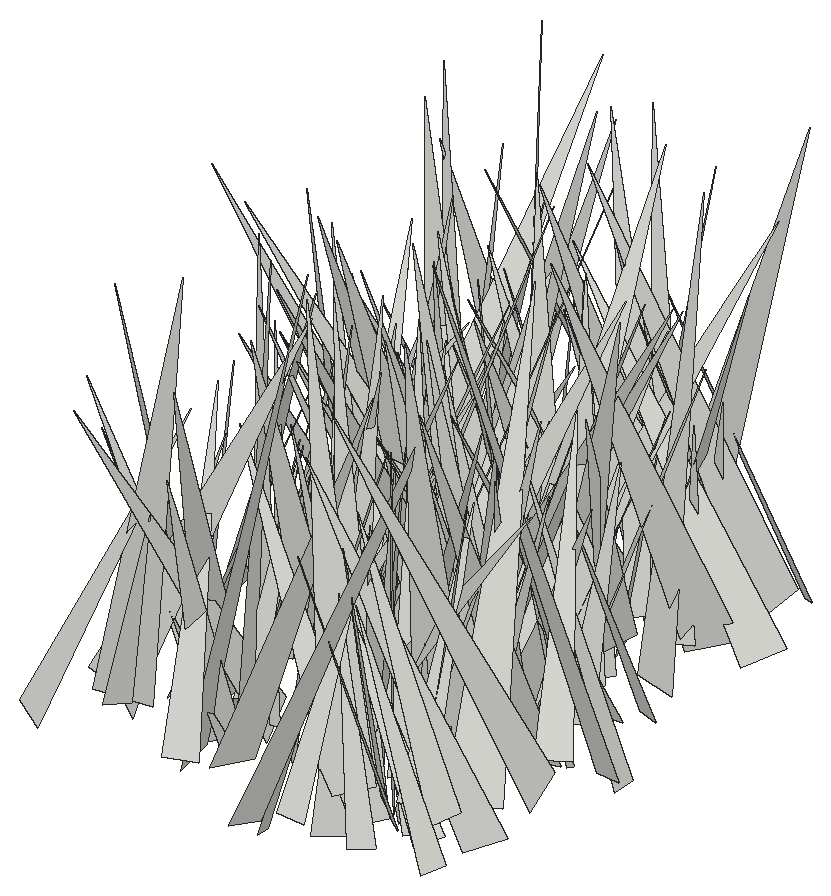
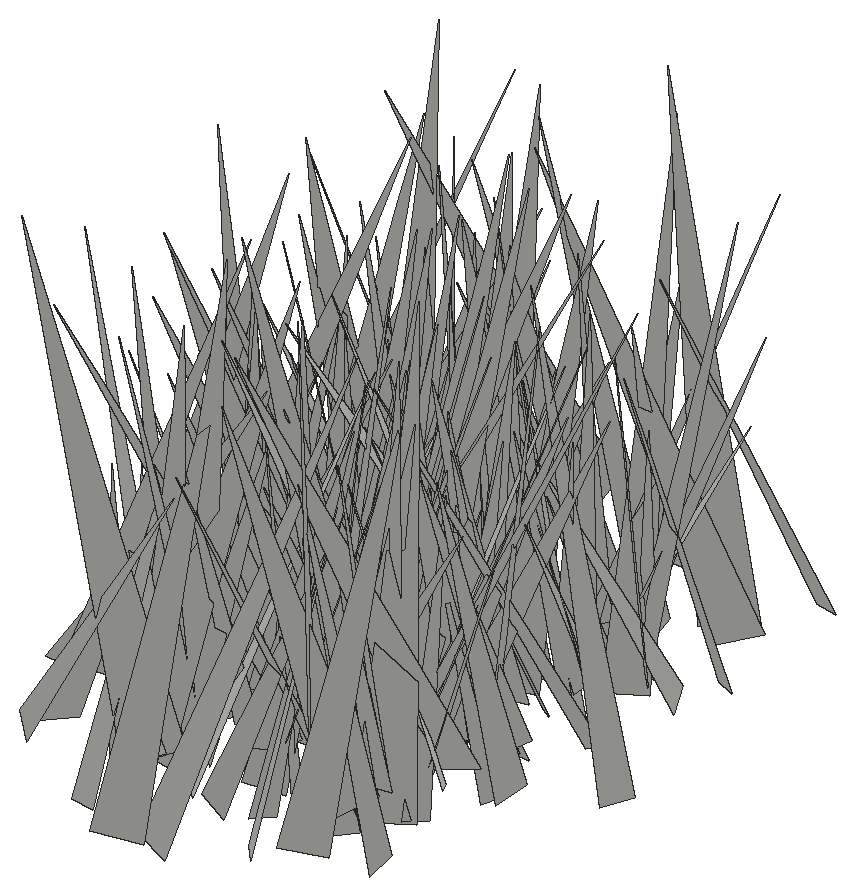
# SketchUp Ruby script. Lengths in inches.
U = 1.inch
M = Sketchup.active_model
def pt(a) = Geom::Point3d.new(a.map { |v| v * U })
def face(e, loops, mat)
  f = e.add_face(loops[0].map { |a| pt(a) })
  loops[1..].each { |l| e.add_face(l.map { |a| pt(a) }).erase! }
  f.material = f.back_material = mat if mat
  f
end
# faces: each face lists its corners as indices into pts; further lists are holes
def faces(e, pts, list, mat = nil) = list.each { |f| face(e, (f[0].is_a?(Array) ? f : [f]).map { |l| l.map { |i| pts[i] } }, mat) }
# xy, xz, yz: faces in a plane at the given z, y or x. An outline is a flat list of corners, or four numbers for a rectangle; further outlines are holes
def ring(l) = l.size == 4 ? [[l[0], l[1]], [l[2], l[1]], [l[2], l[3]], [l[0], l[3]]] : l.each_slice(2).to_a
def flat(e, list, mat, &to3) = list.each { |f| face(e, (f[0].is_a?(Array) ? f : [f]).map { |l| ring(l).map { |u, v| to3.(u, v) } }, mat) }
def xy(e, z, list, mat = nil) = flat(e, list, mat) { |x, y| [x, y, z] }
def xz(e, y, list, mat = nil) = flat(e, list, mat) { |x, z| [x, y, z] }
def yz(e, x, list, mat = nil) = flat(e, list, mat) { |y, z| [x, y, z] }
def lines(e, pts, list) = list.each { |a, b| e.add_line(pt(pts[a]), pt(pts[b])) }
# prism: a flat outline (further loops are holes) pulled along v
def prism(e, loops, v, mat = nil)
  f = face(e, loops, mat); d = Geom::Vector3d.new(v.map { |x| x * U })
  f.pushpull(f.normal.samedirection?(d) ? d.length : -d.length)
end
def box(e, o, s, mat = nil) = prism(e, [[o, [o[0] + s[0], o[1], o[2]], [o[0] + s[0], o[1] + s[1], o[2]], [o[0], o[1] + s[1], o[2]]]], [0, 0, s[2]], mat)
def at(x, y, z, deg = 0) = Geom::Transformation.translation(pt([x, y, z])) * Geom::Transformation.rotation(ORIGIN, Z_AXIS, deg.degrees)
def axes(o, x, y, z) = Geom::Transformation.new([*x, 0, *y, 0, *z, 0, *pt(o).to_a, 1])
def part(name) = M.definitions.add(name)
# library, detail: a bought-in or finely detailed component or shape, given as its bounding box
def library(name, o, s) = part(name).tap { |d| box(d.entities, o, s) }
def detail(e, o, s) = box(e.add_group.entities, o, s)
def put(e, d, t, mat = nil) = e.add_instance(d, t).tap { |i| i.material = mat if mat }
def group(e, t, mat = nil) = e.add_group.tap { |g| g.transformation = t; g.material = mat if mat }.entities
root = M.entities
c1 = part("fur_instance\#9")
p = [[0.8125,0,1.79],[0.67,-0.02,1.48],[0,-0.11,0],[0,0.11,0]]
faces(c1.entities,p,[[0,1,2,3]])
put(root,c1,axes([126.4,82.98,-27.1],[-4.21104,-1.2398,0.43934],[-1.31531,3.95873,-1.43574],[-0.00925,1.50143,4.14832]))
put(root,c1,axes([122.02,80.37,-28.22],[7.393,0.04175,0.28729],[0.1077,-7.1937,-1.72622],[-0.26959,-1.72907,7.18877]))
put(root,c1,axes([126.64,73.74,-27.1],[-5.33847,-0.05884,0.40473],[-0.0096,5.31499,0.64603],[0.40887,-0.64342,5.29956]))
put(root,c1,axes([125.85,74.4,-27.1],[-3.47477,-5.64058,1.59223],[-5.83486,3.50381,-0.32112],[0.55295,1.52727,6.61718]))
put(root,c1,axes([123.08,69.83,-27.1],[2.64419,5.03318,0.33977],[4.95036,-2.51506,-1.26831],[0.97076,-0.88412,5.54221]))
put(root,c1,axes([124.5,76.02,-27.1],[3.53151,3.08583,1.68165],[3.37882,-3.63698,-0.42174],[-0.96639,-1.43941,4.67077]))
put(root,c1,axes([123.76,73.4375,-28.22],[2.7927,4.03544,0.85961],[4.11922,-2.66751,-0.85986],[0.23622,-1.19268,4.83163]))
put(root,c1,axes([124.58,81.87,-28.22],[5.08359,-0.28901,1.82683],[-0.68576,-5.25683,1.07667],[-1.71772,1.24337,4.97667]))
put(root,c1,axes([127.85,83.42,-28.22],[-8.04638,-2.10125,0.20494],[-2.02323,7.90531,1.61682],[0.60315,-1.51404,8.15753]))
put(root,c1,axes([124.33,74.79,-28.22],[4.4552,2.25801,0.37031],[2.04407,-4.29173,1.57715],[-1.02836,1.2518,4.7392]))
put(root,c1,axes([127.79,73.02,-28.22],[-4.47703,-2.46915,0.00102],[-2.34184,4.24552,-1.62229],[-0.78262,1.42103,4.84857]))
put(root,c1,axes([125.86,81.34,-28.22],[-6.04607,-3.24149,2.31572],[-3.3744,6.40425,0.15438],[2.11738,0.95032,6.85845]))
put(root,c1,axes([125.81,76.18,-28.22],[3.59429,3.23742,0.8797],[2.57384,-3.488,2.32011],[-2.15177,1.23558,4.24464]))
put(root,c1,axes([126.67,76.94,-27.1],[1.26657,4.59176,1.22685],[4.36989,-1.62436,1.56816],[-1.86909,-0.68616,4.4977]))
put(root,c1,axes([126.86,81.64,-27.1],[0.11807,-5.18176,0.38422],[-4.95689,-0.22756,-1.54584],[-1.55804,0.33133,4.94722]))
put(root,c1,axes([125.82,89.55,-27.1],[3.87648,-5.20572,1.47803],[-5.00062,-4.14086,-1.46909],[-2.0683,0.2548,6.32205]))
put(root,c1,axes([124.22,78.45,-27.1],[2.61371,2.45973,0.53308],[2.49517,-2.43181,-1.01309],[0.32949,-1.09634,3.44317]))
put(root,c1,axes([124.6875,71.85,-27.1],[2.97768,-2.23657,0.59018],[-2.29034,-2.98547,0.24174],[-0.32391,0.5494,3.71623]))
put(root,c1,axes([124.91,81.26,-27.1],[3.82826,-1.89723,1.31218],[-2.241,-3.66166,1.2438],[-0.54703,1.72325,4.08754]))
put(root,c1,axes([127.42,75.15,-28.22],[1.80048,6.74236,1.9451],[6.61582,-2.30046,1.85022],[-2.33959,-1.31645,6.72888]))
put(root,c1,axes([125.53,77.95,-27.1],[4.20313,-0.16718,1.34956],[-0.39887,-4.34286,0.70427],[-1.30006,0.79192,4.14708]))
put(root,c1,axes([127.31,83.125,-28.22],[1.43774,-5.64122,0.58152],[-5.34924,-1.54822,-1.79367],[-1.88339,0.09091,5.53834]))
put(root,c1,axes([125.81,74.35,-28.22],[0.22689,-3.51122,0.97081],[-3.62685,-0.12635,0.39066],[0.3422,0.98893,3.49679]))
put(root,c1,axes([124.82,82.47,-28.22],[3.6641,-0.22277,0.06955],[-0.2117,-3.63329,-0.48425],[-0.09821,-0.47926,3.63879]))
put(root,c1,axes([126.34,85.27,-28.22],[-4.81324,5.46383,3.73935],[6.29264,5.21276,0.48307],[2.05886,-3.15867,7.26549]))
put(root,c1,axes([126.35,75.01,-28.22],[3.32895,2.2471,0.95718],[1.81279,-3.35751,1.57751],[-1.63691,0.85163,3.69362]))
put(root,c1,axes([126.71,84.79,-27.1],[3.29752,4.92899,1.52703],[4.76096,-3.60504,1.35547],[-1.98997,-0.45731,5.77332]))
put(root,c1,axes([124.9,87.24,-28.22],[5.83146,1.27805,1.15338],[1.33487,-5.92923,-0.17895],[-1.08712,-0.42484,5.96719]))
put(root,c1,axes([124.6,72.21,-27.1],[3.42079,-7.2545,1.9343],[-7.49487,-3.17419,1.34998],[0.44283,2.31686,7.90614]))
put(root,c1,axes([125.74,84.65,-28.22],[4.34393,-1.36952,0.92271],[-1.07858,-4.31928,-1.3331],[-1.25046,-1.03195,4.35524]))
put(root,c1,axes([123.1875,79.92,-27.1],[2.725,5.40327,0.30402],[4.86473,-2.29653,-2.78814],[2.3711,-1.498,5.37096]))
put(root,c1,axes([128.18,83.05,-28.22],[1.43872,7.93621,2.15807],[7.82752,-1.99366,2.11323],[-2.52399,-1.65906,7.7838]))
put(root,c1,axes([127.54,75.52,-28.22],[-6.83742,-2.67371,1.15288],[-1.91772,6.34944,3.35188],[2.19094,-2.7864,6.53176]))
put(root,c1,axes([127.33,82.94,-27.1],[-4.17954,-4.03403,0.06779],[-3.83281,4.00041,1.74723],[1.26,-1.21235,5.53978]))
put(root,c1,axes([125.35,77.76,-28.22],[4.61843,1.91697,0.98697],[2.11588,-4.47821,-1.2031],[-0.41467,-1.49987,4.85358]))
put(root,c1,axes([129.0625,85.36,-28.22],[-2.08811,-4.65792,0.59921],[-4.45757,1.75934,-1.85749],[-1.47829,1.27435,4.7546]))
put(root,c1,axes([126.12,80.45,-28.22],[4.29417,-2.87763,1.75823],[-3.19183,-4.38696,0.6155],[-1.08829,1.5119,5.13243]))
put(root,c1,axes([128.73,83.49,-28.22],[-4.60264,5.20733,0.96805],[5.29634,4.53648,0.77902],[0.04773,-1.24166,6.90606]))
put(root,c1,axes([125.53,83.28,-27.1],[-1.37451,8.097,0.63904],[7.82187,1.49419,-2.10823],[2.18815,-0.25501,7.93763]))
put(root,c1,axes([128.39,80.29,-27.1],[-5.1626,-2.88411,0.4563],[-2.82641,5.16852,0.6903],[0.7333,-0.3834,5.87316]))
put(root,c1,axes([125.05,84.25,-27.1],[3.85978,2.30102,0.3483],[2.28006,-3.60384,-1.45862],[0.46617,-1.42533,4.2503]))
put(root,c1,axes([126.92,84.42,-28.22],[3.98276,-1.20965,1.22676],[-0.42908,-3.68899,-2.24451],[-1.66855,-1.93873,3.5054]))
put(root,c1,axes([126.39,85.42,-27.1],[0.00091,-3.67707,1.93886],[-4.08733,0.35251,0.67045],[0.75747,1.90654,3.61543]))
put(root,c1,axes([123.86,72.64,-27.1],[0.25719,7.17904,2.90731],[6.91163,1.10018,-3.3281],[3.49578,-2.70337,6.36621]))
put(root,c1,axes([126.95,80.76,-27.1],[-5.68198,1.58826,2.45655],[1.00817,6.10119,-1.61279],[2.74605,1.04639,5.67506]))
put(root,c1,axes([128.11,70.43,-27.1],[-0.8094,5.47668,0.09308],[5.43232,0.79056,0.72297],[-0.70181,-0.19701,5.48875]))
put(root,c1,axes([127.39,87.04,-27.1],[6.18055,4.14964,3.19418],[4.26505,-6.85588,0.65402],[-3.03836,-1.18276,7.41558]))
put(root,c1,axes([127.93,73.5625,-28.22],[-6.64988,-1.58039,2.79885],[-2.32051,6.81074,-1.66765],[2.22405,2.38079,6.62853]))
put(root,c1,axes([128.15,77.76,-28.22],[-1.83957,6.80237,0.25254],[6.80704,1.83779,0.08208],[-0.01336,-0.2652,7.04624]))
put(root,c1,axes([128.04,77.9,-28.22],[-5.21181,1.32812,1.31914],[0.83689,5.14396,-1.87252],[1.67442,1.56295,5.04188]))
put(root,c1,axes([127.82,85.5,-27.1],[-5.63617,-2.55407,1.20627],[-1.85262,5.37498,2.72438],[2.13217,-2.08115,5.55585]))
put(root,c1,axes([125.6875,75.45,-28.22],[7.80685,-2.34529,0.78759],[-1.91376,-7.37702,-2.99744],[-1.56786,-2.67335,7.58041]))
put(root,c1,axes([127.01,73.67,-28.22],[4.0127,-3.86264,0.72099],[-3.71726,-4.06564,-1.09277],[-1.27351,-0.30356,5.46147]))
put(root,c1,axes([126.24,86.68,-27.1],[6.10707,-2.19869,2.10682],[-2.76305,-5.98564,1.76265],[-1.28003,2.43046,6.24689]))
put(root,c1,axes([126.83,86.52,-28.22],[2.82245,-3.27125,1.23973],[-3.47956,-2.78972,0.56063],[-0.36142,1.31172,4.28404]))
put(root,c1,axes([127.43,74.34,-27.1],[-2.50227,2.59124,1.1484],[2.47228,2.74461,-0.80603],[1.38608,-0.21748,3.51087]))
put(root,c1,axes([128.72,78.55,-27.1],[-0.54656,4.2534,1.19948],[4.32093,0.26075,1.04426],[-0.92722,-1.29209,4.15928]))
put(root,c1,axes([129.91,76.66,-28.22],[-7.28792,0.99409,0.70676],[0.80322,7.1337,-1.75122],[0.9179,1.65037,7.1439]))
put(root,c1,axes([128.19,88.93,-28.22],[-3.7934,-3.57067,0.95546],[-3.47781,3.9116,0.81037],[1.25196,0.04698,5.14615]))
put(root,c1,axes([127.72,82.61,-27.1],[0.59961,-8.00132,0.48644],[-8.01433,-0.60861,-0.13198],[-0.1682,0.47514,8.02267]))
put(root,c1,axes([126.53,81.82,-27.1],[-1.2496,-4.95098,2.04852],[-4.91628,1.89585,1.58307],[2.13046,1.47094,4.85465]))
put(root,c1,axes([129.07,79.91,-28.22],[-2.83398,-2.56318,0.53676],[-2.6174,2.79801,-0.45803],[0.08496,0.70049,3.79362]))
put(root,c1,axes([125.68,80.01,-28.22],[2.98745,4.37857,0.43851],[4.21633,-2.69647,-1.80015],[1.25963,-1.35874,4.98559]))
put(root,c1,axes([131,81.97,-27.1],[-8.10416,-1.22815,0.06312],[-1.16757,7.81624,2.17553],[0.38615,-2.14192,7.90272]))
put(root,c1,axes([128.11,82.85,-28.22],[5.75232,0.0292,2.58276],[0.25276,-6.28131,-0.49192],[-2.57052,-0.55229,5.73133]))
put(root,c1,axes([128.32,77.18,-28.22],[2.5513,-6.67742,1.15565],[-6.68995,-2.67869,-0.70836],[-1.08074,0.81812,7.11304]))
put(root,c1,axes([128.88,83.57,-28.22],[-6.19203,-3.31038,1.54754],[-2.85802,6.28451,2.00782],[2.2771,-1.114,6.72819]))
put(root,c1,axes([129.36,81.83,-28.22],[-4.79801,0.15244,1.14259],[0.25589,4.91001,0.4195],[1.12396,-0.46714,4.78206]))
put(root,c1,axes([127.09,72.32,-28.22],[7.84011,2.17766,1.89393],[2.14429,-8.06482,0.39652],[-1.93163,-0.114,8.12726]))
put(root,c1,axes([129.16,87.13,-28.22],[-3.50463,1.38607,1.3282],[1.66931,3.56562,0.68373],[0.94799,-1.15452,3.70623]))
put(root,c1,axes([129.59,82.98,-27.1],[-4.54367,3.48057,1.82928],[3.81076,4.58683,0.73803],[0.96889,-1.71821,5.67579]))
put(root,c1,axes([128.3,82.45,-27.1],[6.29678,-5.28708,1.00032],[-4.88133,-6.26054,-2.36253],[-2.26416,-1.20654,7.87535]))
put(root,c1,axes([126.65,84.53,-27.1],[3.7348,-2.45498,0.02516],[-2.33086,-3.53122,1.44009],[0.77113,1.21649,4.23106]))
put(root,c1,axes([130.01,75.8125,-27.1],[-1.05409,-4.02831,1.60299],[-4.27873,0.70037,-1.05356],[-0.69957,1.78611,4.02845]))
put(root,c1,axes([130.61,87.53,-28.22],[-1.8038,-4.78632,0.84713],[-4.75617,1.55162,-1.36069],[-1.00264,1.25053,4.93062]))
put(root,c1,axes([126.75,77.63,-28.22],[3.37481,3.69249,0.11879],[3.55193,-3.19874,-1.47981],[1.01606,-1.08238,4.77849]))
put(root,c1,axes([128.71,79.71,-27.1],[0.78552,4.64999,1.51438],[4.88897,-0.70993,-0.35606],[0.11721,-1.55126,4.70241]))
put(root,c1,axes([130.53,90.34,-28.22],[-3.40543,-6.99905,0.02732],[-6.9991,3.40539,-0.01642],[-0.00281,0.03175,7.78353]))
put(root,c1,axes([130.52,85.77,-27.1],[-4.35819,2.96505,1.59627],[3.3258,4.19926,1.28011],[0.52792,-1.97688,5.11338]))
put(root,c1,axes([126.78,85.93,-28.22],[2.90433,5.023,0.38727],[4.82562,-2.64532,-1.87916],[1.44702,-1.25991,5.48948]))
put(root,c1,axes([130.23,84.67,-27.1],[-3.91317,-2.34388,0.53173],[-2.28614,3.94348,0.55853],[0.74167,-0.21123,4.52711]))
put(root,c1,axes([127.4375,82.21,-28.22],[6.75975,3.62956,0.52461],[3.54067,-6.74583,1.04905],[-0.95528,0.68056,7.60048]))
put(root,c1,axes([126.79,79.36,-28.22],[6.15209,3.35933,0.33959],[3.37614,-6.1107,-0.71393],[0.04606,-0.78923,6.97306]))
put(root,c1,axes([127.47,84.39,-27.1],[7.2049,-3.47591,1.96261],[-3.83046,-7.15988,1.38131],[-1.1231,2.12096,7.87937]))
put(root,c1,axes([128.47,79.41,-28.22],[-0.37702,3.57753,2.02822],[3.88687,0.97529,-0.99777],[1.34335,-1.81786,3.4562]))
put(root,c1,axes([132.25,73.05,-28.22],[-2.56552,5.11443,0.44811],[4.78646,2.20153,2.27666],[-1.85689,-1.39139,5.24939]))
put(root,c1,axes([130.89,80.43,-27.1],[0.06912,-7.57158,0.2529],[-7.42195,-0.11839,-1.51598],[-1.51902,0.23392,7.41859]))
put(root,c1,axes([129.16,80.94,-28.22],[-1.69129,6.09931,0.73665],[6.01995,1.79783,-1.06428],[1.22654,-0.41345,6.23934]))
put(root,c1,axes([128.9,84.78,-27.1],[-3.46675,-5.54657,1.13696],[-5.08588,3.63649,2.23277],[2.48816,-0.29493,6.14797]))
put(root,c1,axes([128.1,76.6,-28.22],[6.40795,-1.734,1.03011],[-1.73088,-6.48917,-0.15614],[-1.03535,0.11648,6.63658]))
put(root,c1,axes([129.17,74.13,-28.22],[-4.33935,-4.28478,3.74469],[-5.00881,5.11096,0.04388],[2.70071,2.59437,6.09815]))
put(root,c1,axes([130.02,79.4,-27.1],[-3.10303,1.40825,1.48641],[1.65077,3.31728,0.3033],[1.21143,-0.91317,3.39411]))
put(root,c1,axes([130.86,81.93,-27.1],[-4.62696,-2.40171,1.71965],[-2.7299,4.69747,-0.78458],[1.12828,1.51649,5.15378]))
put(root,c1,axes([130.14,85.84,-28.22],[1.50349,-5.86365,0.5049],[-5.82358,-1.55753,-0.74685],[-0.85041,0.2992,6.00709]))
put(root,c1,axes([129.38,85.36,-28.22],[4.70905,2.28139,1.77217],[2.5251,-4.89691,-0.40574],[-1.40329,-1.15586,5.21682]))
put(root,c1,axes([130.57,80.94,-27.1],[4.49335,-4.83843,2.48866],[-4.8443,-5.0271,-1.02712],[-2.47721,1.05444,6.5227]))
put(root,c1,axes([129.81,76.22,-27.1],[5.70548,5.18554,0.14342],[4.71826,-5.27598,3.06024],[-2.15603,2.1765,7.07653]))
put(root,c1,axes([131.14,83.21,-28.22],[-5.69,4.35692,2.08043],[4.49689,5.95288,-0.16772],[1.75752,-1.1258,7.16454]))
put(root,c1,axes([131.9,78.12,-28.22],[-4.58656,-0.99691,0.53395],[-0.9871,4.61746,0.14195],[0.55187,-0.02624,4.69151]))
put(root,c1,axes([128.16,72.74,-28.22],[6.91635,-1.96319,0.7746],[-2.05636,-6.86586,0.95992],[-0.47486,1.1384,7.12521]))
put(root,c1,axes([131.43,73.69,-28.22],[-5.3119,3.70536,1.5571],[3.75007,5.49761,-0.28937],[1.44609,-0.64586,6.4701]))
put(root,c1,axes([131.67,87.17,-28.22],[-4.86076,-4.47494,0.06756],[-4.36579,4.76306,1.38194],[0.98465,-0.972,6.46083]))
put(root,c1,axes([130.2,80.85,-27.1],[2.51881,-4.55482,0.15905],[-4.51842,-2.51942,-0.59372],[-0.59628,-0.14918,5.17091]))
put(root,c1,axes([131.42,81.3,-27.1],[-3.70308,-3.24105,0.05421],[-3.08159,3.54543,1.46762],[1.00557,-1.07036,4.69716]))
put(root,c1,axes([130.99,79.5,-27.1],[5.55902,-2.83125,1.90418],[-2.404,-5.83322,-1.65498],[-2.42129,-0.70867,6.01496]))
put(root,c1,axes([132.05,80.81,-28.22],[-3.13044,2.30171,0.23571],[2.28042,3.13636,-0.34054],[0.39127,0.13578,3.8706]))
put(root,c1,axes([132.06,80.46,-28.22],[-5.09295,0.86723,1.4086],[1.03106,5.23004,0.50795],[1.29351,-0.75432,5.14123]))
put(root,c1,axes([130.69,82.13,-28.22],[4.01363,-0.60213,1.19124],[-0.70216,-4.16285,0.26162],[-1.13516,0.446,4.0501]))
put(root,c1,axes([133.38,76.06,-27.1],[-5.0928,-0.09663,0.30052],[-0.16718,4.94609,-1.24277],[0.26777,1.25023,4.93978]))
put(root,c1,axes([133.03,71.29,-28.22],[-7.41355,2.38035,1.13819],[1.92535,7.2016,-2.52036],[1.80404,2.09598,7.36713]))
put(root,c1,axes([131.31,70.2,-28.22],[5.08694,2.79276,1.06084],[2.31416,-5.00849,2.08845],[-1.88933,1.38471,5.41433]))
put(root,c1,axes([131.16,75.84,-27.1],[-1.15878,-4.12917,1.68532],[-4.31214,1.48176,0.66553],[1.13832,1.40977,4.23673]))
put(root,c1,axes([132.6875,86.62,-28.22],[-0.18696,-5.47828,1.21386],[-5.53827,-0.01495,-0.92048],[-0.90141,1.22808,5.40363]))
put(root,c1,axes([133.26,72.3125,-28.22],[-7.28379,2.71503,1.56111],[2.64145,7.44897,-0.63058],[1.68261,0.05921,7.74773]))
put(root,c1,axes([131.36,85.01,-27.1],[0.22863,4.55848,1.01522],[4.65358,-0.13679,-0.43379],[0.39321,-1.03161,4.54355]))
put(root,c1,axes([130.28,81.31,-28.22],[5.40312,-1.02873,0.51523],[-0.87968,-5.28821,-1.33359],[-0.74156,-1.2223,5.33606]))
put(root,c1,axes([132.66,75.38,-28.22],[-5.28353,4.19242,1.51467],[4.2139,5.46353,-0.42331],[1.45386,-0.59977,6.73148]))
put(root,c1,axes([131.58,90.55,-28.22],[2.52782,-6.77606,0.30453],[-6.73549,-2.54598,-0.74076],[-0.80053,0.02468,7.19418]))
put(root,c1,axes([133.25,87.07,-27.1],[1.43067,-7.01564,1.7352],[-6.90944,-1.84641,-1.76845],[-2.11892,1.28394,6.9382]))
put(root,c1,axes([133.02,71.92,-27.1],[-6.40886,3.74132,2.19702],[3.96061,6.64492,0.23769],[1.77143,-1.32114,7.41717]))
put(root,c1,axes([129.9,81.96,-28.22],[5.44846,0.74036,0.07595],[0.73692,-5.44519,0.21553],[-0.10422,0.20337,5.4943]))
put(root,c1,axes([130.36,79.96,-28.22],[5.36031,4.39922,1.5205],[4.6383,-5.24227,-1.18439],[-0.38885,-1.88772,6.83252]))
put(root,c1,axes([130.97,82.1,-27.1],[1.98838,-4.24744,1.75797],[-4.57109,-1.62434,1.24561],[0.4862,2.09896,4.52138]))
put(root,c1,axes([133.4,85.47,-27.1],[-5.88987,4.84378,2.23578],[5.14185,6.04195,0.45575],[1.42207,-1.78441,7.61217]))
put(root,c1,axes([129.79,80.18,-27.1],[0.86928,6.52033,1.58307],[6.24969,-0.2059,-2.58369],[2.44176,-1.79425,6.04937]))
put(root,c1,axes([132.86,78.89,-28.22],[1.6386,-6.2759,2.07036],[-6.47654,-1.94928,-0.78297],[-1.31443,1.78093,6.43885]))
put(root,c1,axes([134.79,72.87,-28.22],[-0.96186,4.58475,0.31518],[4.19254,0.74357,1.97843],[-1.88199,-0.68675,4.24628]))
put(root,c1,axes([130.18,78.65,-27.1],[6.41369,-0.07562,0.05633],[-0.05586,-6.13403,-1.87481],[-0.07597,-1.87412,6.13403]))
put(root,c1,axes([132.36,80.59,-27.1],[-3.86216,7.0455,1.20437],[6.7899,4.04407,-1.88376],[2.2331,-0.11104,7.81068]))
put(root,c1,axes([131.07,82.9375,-27.1],[0.51844,5.23573,1.343],[5.13497,-0.0558,-1.76472],[1.68777,-1.43851,4.95655]))
put(root,c1,axes([134.84,84.42,-27.1],[-0.02832,7.80203,1.3013],[7.5934,-0.33756,2.1891],[-2.2148,-1.25708,7.48868]))
put(root,c1,axes([132.62,84.88,-28.22],[6.22186,3.72093,2.03459],[3.43335,-6.54009,1.46143],[-2.48938,0.27987,7.10078]))
put(root,c1,axes([132.68,69.71,-27.1],[-0.04754,4.40868,0.34675],[4.41199,0.07095,-0.29716],[0.30179,-0.34273,4.39891]))
put(root,c1,axes([133.07,82.91,-28.22],[4.8811,-3.48072,2.77846],[-3.79933,-5.40519,-0.09683],[-2.32386,1.52607,5.99426]))
put(root,c1,axes([132.07,74.48,-27.1],[4.60045,-1.39498,0.802],[-1.20201,-4.59424,-1.0961],[-1.06973,-0.83684,4.68067]))
put(root,c1,axes([131.72,79.43,-28.22],[6.47636,2.00005,0.90058],[1.74291,-6.39683,1.67254],[-1.33173,1.35459,6.56857]))
put(root,c1,axes([134.95,81.49,-28.22],[-1.88046,-5.21634,0.33238],[-5.10911,1.75978,-1.28722],[-1.10347,0.74146,5.39346]))
put(root,c1,axes([130.61,81.53,-27.1],[6.21247,-1.9108,0.54363],[-1.98453,-5.88708,1.9863],[0.09123,2.05733,6.18874]))
put(root,c1,axes([129.75,80.95,-28.22],[7.15691,-3.14413,0.26361],[-3.09126,-6.8566,2.14652],[0.63178,2.06831,7.5166]))
put(root,c1,axes([132.48,80.89,-28.22],[0.96645,3.75371,0.08435],[3.72936,-0.9496,-0.47076],[0.43512,-0.19848,3.84744]))
put(root,c1,axes([132.24,74.18,-28.22],[5.81902,2.09502,1.94943],[2.48849,-5.88572,-1.1028],[-1.4131,-1.7377,6.08555]))
put(root,c1,axes([134.1,71.18,-28.22],[-1.64307,3.38565,0.94063],[3.51296,1.55882,0.52563],[-0.08077,-1.0745,3.72639]))
put(root,c1,axes([130.52,83.16,-28.22],[2.72489,7.5123,0.23605],[7.26372,-2.56761,-2.13568],[1.931,-0.94238,7.70056]))
put(root,c1,axes([133.35,75.05,-28.22],[-0.96334,-4.21277,1.52504],[-4.43315,1.12201,0.29911],[0.64835,1.41239,4.31115]))
put(root,c1,axes([131.85,68.68,-27.1],[7.63616,1.08232,1.22596],[0.61242,-7.3209,2.64853],[-1.51635,2.49367,7.24345]))
put(root,c1,axes([135.38,72.67,-28.22],[-3.19624,2.75407,0.40141],[2.73336,2.9911,1.24258],[-0.52417,-1.19599,4.03198]))
put(root,c1,axes([134.84,77.68,-28.22],[-3.66432,1.46778,0.50332],[1.5223,3.65057,0.437],[0.30055,-0.59495,3.9231]))
put(root,c1,axes([134.17,72.14,-27.1],[-2.56443,-3.19615,1.19823],[-3.34404,2.653,-0.08027],[0.6845,0.98675,4.09698]))
put(root,c1,axes([133.51,89.68,-28.22],[-2.90473,-5.90083,0.221],[-5.68544,2.86131,1.67173],[1.5951,-0.54696,6.36102]))
put(root,c1,axes([136.29,88.79,-27.1],[-3.48224,-3.77241,0.29956],[-3.58403,3.15695,-1.90663],[-1.21472,1.49981,4.76674]))
put(root,c1,axes([135.26,71.25,-27.1],[-2.96371,-3.18096,0.56073],[-3.21747,2.84043,-0.89238],[-0.28422,1.01488,4.25508]))
put(root,c1,axes([132.97,74.04,-28.22],[-4.22534,-4.50008,2.6097],[-4.33201,4.90527,1.44456],[2.88009,0.77613,6.00146]))
put(root,c1,axes([134.47,80.77,-27.1],[-5.32179,3.05618,1.70346],[3.04909,5.5718,-0.47069],[1.71611,-0.42222,6.11884]))
put(root,c1,axes([132.93,80.66,-28.22],[4.24517,2.47398,0.29086],[2.34061,-4.15824,1.20716],[-0.85248,0.90284,4.76286]))
put(root,c1,axes([137.39,85.39,-27.1],[-4.14935,5.21761,0.66717],[4.85978,3.47746,3.02911],[-2.01273,-2.35998,5.93844]))
put(root,c1,axes([135.82,87.89,-27.1],[-7.8024,0.71377,1.7229],[1.19599,7.6017,2.26696],[1.43089,-2.46171,7.49986]))
put(root,c1,axes([135.8,78.58,-28.22],[-3.59352,-1.36236,0.30323],[-1.35819,3.22059,-1.62619],[-0.32136,1.6227,3.48208]))
put(root,c1,axes([136.74,73.51,-28.22],[-3.6368,4.97548,2.15784],[5.29036,2.68314,2.72961],[-1.1932,-3.26854,5.52548]))
put(root,c1,axes([129.79,75.65,-28.22],[5.88193,4.68919,0.48239],[4.10623,-4.71789,-4.20698],[2.31519,-3.54559,6.23594]))
put(root,c1,axes([133.1,88.25,-28.22],[0.93641,-4.49496,0.58968],[-4.44892,-0.79539,1.00188],[0.87152,0.76939,4.48082]))
put(root,c1,axes([133.57,75.65,-27.1],[4.47344,-6.57845,1.38646],[-6.62258,-4.59864,-0.45163],[-1.15746,0.88686,7.94253]))
put(root,c1,axes([132.38,80.3,-28.22],[3.4493,-3.36014,0.02886],[-3.29462,-3.37365,0.97621],[0.66096,0.719,4.71542]))
put(root,c1,axes([132.33,87.96,-27.1],[6.94828,-4.27135,1.74082],[-4.55894,-6.83788,1.41876],[-0.70067,2.13364,8.03182]))
put(root,c1,axes([133.73,73.28,-28.22],[3.70568,3.40586,0.49894],[3.35111,-3.73706,0.62078],[-0.78668,0.12425,4.99466]))
put(root,c1,axes([134.39,80.37,-27.1],[-1.58112,-4.73276,0.31075],[-4.65779,1.61119,0.83937],[0.89473,0.02406,4.91878]))
put(root,c1,axes([136.16,72.42,-27.1],[-4.59292,1.38597,0.57425],[1.45174,4.5724,0.57548],[0.37836,-0.71958,4.76284]))
put(root,c1,axes([133.49,78.78,-27.1],[5.23051,-1.10724,0.78196],[-0.81536,-5.06,-1.7109],[-1.08287,-1.53819,5.06527]))
put(root,c1,axes([133.65,83.44,-27.1],[4.86782,-2.47433,0.4659],[-2.27673,-4.75873,-1.48527],[-1.07512,-1.1257,5.25471]))
put(root,c1,axes([134.73,83.76,-28.22],[2.04699,7.14679,2.15899],[7.40344,-2.23185,0.36858],[-0.96272,-1.9673,7.42502]))
put(root,c1,axes([134.29,76.6,-27.1],[3.78689,-0.0231,1.24793],[-0.32688,-3.86581,0.92039],[-1.20458,0.97644,3.67342]))
put(root,c1,axes([134.39,80.64,-28.22],[-2.57998,2.99071,1.64125],[3.02202,2.95835,-0.64026],[1.58287,-0.77341,3.89753]))
put(root,c1,axes([134.34,85.96,-27.1],[-0.14412,-3.47359,1.04669],[-3.58722,0.2928,0.47779],[0.54152,1.01518,3.44359]))
put(root,c1,axes([134.09,74.8,-28.22],[4.78963,3.34115,0.62659],[3.09789,-4.73577,1.57225],[-1.39963,0.95165,5.62422]))
put(root,c1,axes([133.18,81.99,-28.22],[4.74716,3.3592,0.52437],[3.38285,-4.75689,-0.1518],[-0.33985,-0.42721,5.81349]))
put(root,c1,axes([133.65,75.99,-28.22],[5.79665,-1.91222,1.6292],[-2.17494,-5.87047,0.84811],[-1.25719,1.33905,6.04471]))
put(root,c1,axes([134.78,78.22,-28.22],[1.39715,-7.46285,0.32526],[-7.45597,-1.41344,-0.40331],[-0.45656,0.24497,7.58179]))
put(root,c1,axes([136.51,71.45,-28.22],[-3.98782,0.86871,0.11292],[0.87287,3.98492,0.16912],[0.07423,-0.18933,4.07783]))
put(root,c1,axes([135.83,85.05,-27.1],[3.52912,-6.81057,1.30534],[-6.45742,-3.76145,-2.16695],[-2.52774,0.10047,7.35818]))
put(root,c1,axes([132.32,82.97,-27.1],[0.1957,-7.90399,1.09327],[-7.43409,0.21668,2.89722],[2.89871,1.0893,7.35646]))
put(root,c1,axes([134.4,73.72,-27.1],[4.12014,1.91723,1.34742],[2.03951,-4.27599,-0.15214],[-1.154,-0.71202,4.54182]))
put(root,c1,axes([135,72.45,-27.1],[-1.136,4.49998,0.83575],[4.53043,1.22799,-0.4539],[0.65076,-0.69355,4.61891]))
put(root,c1,axes([132.18,87.44,-27.1],[7.41722,0.99885,0.34739],[1.05742,-6.96886,-2.53978],[0.01548,-2.56338,7.04006]))
put(root,c1,axes([138.26,77.19,-27.1],[-4.4516,-6.59475,1.62319],[-6.65602,3.85048,-2.61027],[-1.35017,2.76139,7.51625]))
put(root,c1,axes([135.68,82.24,-28.22],[-1.2303,-3.6424,0.32202],[-3.65502,1.23499,0.00478],[0.10759,0.30356,3.84457]))
put(root,c1,axes([136.42,77.02,-27.1],[-3.1637,4.01487,0.30871],[3.99884,3.17867,-0.35895],[0.47305,-0.01931,5.09895]))
put(root,c1,axes([136.31,73.51,-27.1],[-5.32969,5.59283,1.04722],[5.46672,5.43108,-1.18331],[1.57839,0.07463,7.63447]))
put(root,c1,axes([137.69,78.64,-28.22],[-5.12979,-1.0122,0.11272],[-1.018,5.07872,-0.72273],[-0.03042,0.73083,5.17851]))
put(root,c1,axes([137.34,75.36,-27.1],[-7.29024,-1.74958,0.87658],[-1.40156,7.02793,2.37084],[1.36568,-2.12702,7.11251]))
